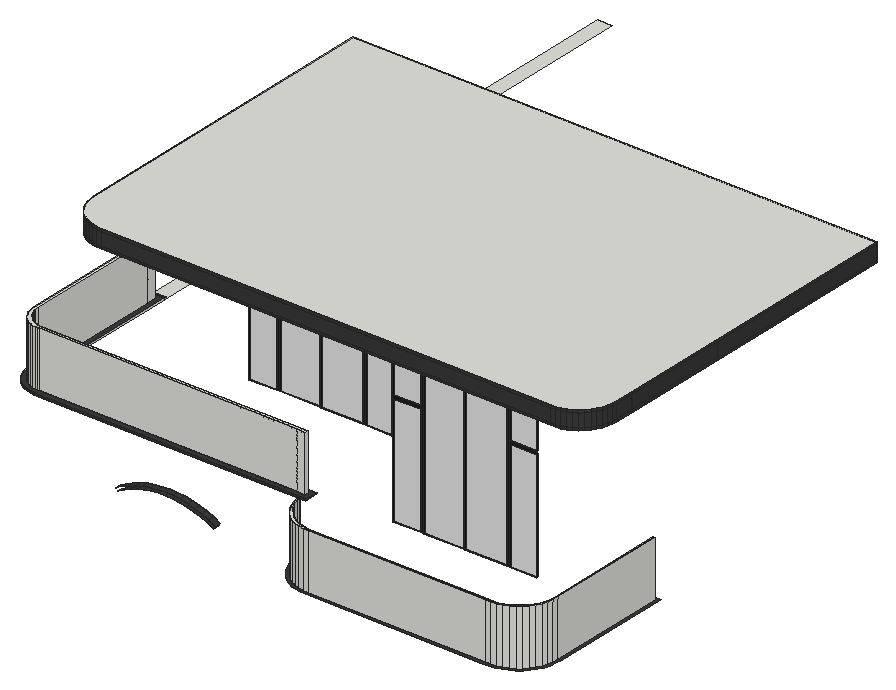
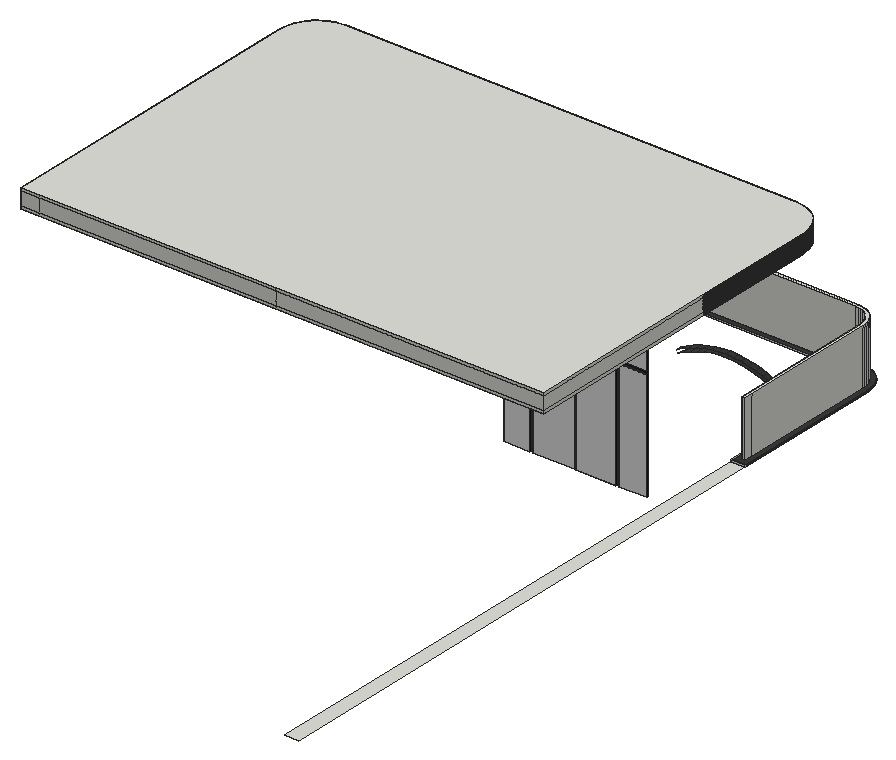
# SketchUp Ruby script. Lengths in inches.
U = 1.inch
M = Sketchup.active_model
def pt(a) = Geom::Point3d.new(a.map { |v| v * U })
def face(e, loops, mat)
  f = e.add_face(loops[0].map { |a| pt(a) })
  loops[1..].each { |l| e.add_face(l.map { |a| pt(a) }).erase! }
  f.material = f.back_material = mat if mat
  f
end
# faces: each face lists its corners as indices into pts; further lists are holes
def faces(e, pts, list, mat = nil) = list.each { |f| face(e, (f[0].is_a?(Array) ? f : [f]).map { |l| l.map { |i| pts[i] } }, mat) }
# xy, xz, yz: faces in a plane at the given z, y or x. An outline is a flat list of corners, or four numbers for a rectangle; further outlines are holes
def ring(l) = l.size == 4 ? [[l[0], l[1]], [l[2], l[1]], [l[2], l[3]], [l[0], l[3]]] : l.each_slice(2).to_a
def flat(e, list, mat, &to3) = list.each { |f| face(e, (f[0].is_a?(Array) ? f : [f]).map { |l| ring(l).map { |u, v| to3.(u, v) } }, mat) }
def xy(e, z, list, mat = nil) = flat(e, list, mat) { |x, y| [x, y, z] }
def xz(e, y, list, mat = nil) = flat(e, list, mat) { |x, z| [x, y, z] }
def yz(e, x, list, mat = nil) = flat(e, list, mat) { |y, z| [x, y, z] }
def lines(e, pts, list) = list.each { |a, b| e.add_line(pt(pts[a]), pt(pts[b])) }
# prism: a flat outline (further loops are holes) pulled along v
def prism(e, loops, v, mat = nil)
  f = face(e, loops, mat); d = Geom::Vector3d.new(v.map { |x| x * U })
  f.pushpull(f.normal.samedirection?(d) ? d.length : -d.length)
end
def box(e, o, s, mat = nil) = prism(e, [[o, [o[0] + s[0], o[1], o[2]], [o[0] + s[0], o[1] + s[1], o[2]], [o[0], o[1] + s[1], o[2]]]], [0, 0, s[2]], mat)
def at(x, y, z, deg = 0) = Geom::Transformation.translation(pt([x, y, z])) * Geom::Transformation.rotation(ORIGIN, Z_AXIS, deg.degrees)
def axes(o, x, y, z) = Geom::Transformation.new([*x, 0, *y, 0, *z, 0, *pt(o).to_a, 1])
def part(name) = M.definitions.add(name)
# library, detail: a bought-in or finely detailed component or shape, given as its bounding box
def library(name, o, s) = part(name).tap { |d| box(d.entities, o, s) }
def detail(e, o, s) = box(e.add_group.entities, o, s)
def put(e, d, t, mat = nil) = e.add_instance(d, t).tap { |i| i.material = mat if mat }
def group(e, t, mat = nil) = e.add_group.tap { |g| g.transformation = t; g.material = mat if mat }.entities
root = M.entities
M.materials.add("[Color M07]").color = [58, 58, 58]
M.materials.add("[Color M08]").color = [30, 30, 30]
M.materials.add("[Mirror 02]").color = [229, 229, 229]
xy(root,265.57,[[216.74,2.48,213.39,2.7,210.15,3.35,207.02,4.41,204.06,5.87,201.31,7.71,198.82,9.89,196.65,12.37,194.81,15.12,193.35,18.08,192.29,21.21,191.64,24.45,191.57,25.58,192.97,25.58,193.03,24.64,193.64,21.57,194.64,18.62,196.02,15.82,197.76,13.22,199.8125,10.875,202.16,8.82,204.76,7.08,207.56,5.7,210.51,4.7,213.57,4.09,216.79,3.88,331.6,3.88,335.01,3.93,338.19,4.4,341.28,5.31,344.22,6.62,346.96,8.3125,349.44,10.36,351.62,12.73,353.46,15.37,354.93,18.23,356,21.26,356.64,24.41,356.87,27.73,356.87,106.25,358.27,106.25,358.27,27.68,358.03,24.23,357.34,20.89,356.21,17.68,354.66,14.64,352.71,11.85,350.4,9.35,347.77,7.18,344.875,5.38,341.77,3.99,338.5,3.04,335.125,2.53,331.61,2.48],[189.6875,27.75,195,27.75,194.98,28.1]])
xy(root,265.57,[[[216.67,0.3125,331.63,0.3125,335.3,0.36,338.96,0.91,342.52,1.95,345.9,3.46,349.04,5.41,351.89,7.77,354.4,10.49,356.52,13.52,358.21,16.82,359.44,20.31,360.1875,23.93,360.4375,27.61,360.4375,108.42,354.7,108.42,354.7,27.8,354.49,24.71,353.9,21.85,352.93,19.09,351.59,16.49,349.92,14.09,347.94,11.94,345.6875,10.08,343.2,8.54,340.53,7.35,337.73,6.53,334.84,6.09,331.59,6.05,216.86,6.05,213.86,6.25,211.07,6.8,208.39,7.71,205.84,8.97,203.48,10.54,201.35,12.41,199.48,14.55,197.91,16.91,196.65,19.45,195.74,22.14,195.1875,24.92,195,27.75,189.6875,27.75,189.25,27.72,189.48,24.17,190.18,20.65,191.34,17.25,192.93,14.03,194.92,11.05,197.29,8.35,199.98,5.98,202.97,3.99,206.1875,2.4,209.59,1.25,213.11,0.55],[216.74,2.48,213.39,2.7,210.15,3.35,207.02,4.41,204.06,5.87,201.31,7.71,198.82,9.89,196.65,12.37,194.81,15.12,193.35,18.08,192.29,21.21,191.64,24.45,191.57,25.58,192.97,25.58,193.03,24.64,193.64,21.57,194.64,18.62,196.02,15.82,197.76,13.22,199.8125,10.875,202.16,8.82,204.76,7.08,207.56,5.7,210.51,4.7,213.57,4.09,216.79,3.88,331.6,3.88,335.01,3.93,338.19,4.4,341.28,5.31,344.22,6.62,346.96,8.3125,349.44,10.36,351.62,12.73,353.46,15.37,354.93,18.23,356,21.26,356.64,24.41,356.87,27.73,356.87,106.25,358.27,106.25,358.27,27.68,358.03,24.23,357.34,20.89,356.21,17.68,354.66,14.64,352.71,11.85,350.4,9.35,347.77,7.18,344.875,5.38,341.77,3.99,338.5,3.04,335.125,2.53,331.61,2.48]]],"[Color M07]")
xy(root,266.52,[[205.38,85.4375,223.05,86.25],[225.05,85.4375,250.97,86.25],[251.97,85.4375,278.89,86.25],[280.89,85.4375,298.16,86.25],[56.75,154.4375,74.42,155.25],
  [76.42,154.4375,102.34,155.25],[103.34,154.4375,130.27,155.25],[132.27,154.4375,149.53,155.25]],"[Color M08]")
xy(root,300,[[0,145.57,9,146.28],[0,146.28,9,507.75]])
xy(root,301.0625,[[18.77,31.13,16.92,31.25,14.92,31.65,12.99,32.3,11.16,33.21,9.47,34.34,7.93,35.68,6.59,37.22,5.46,38.91,4.55,40.74,3.9,42.67,3.5,44.67,3.38,46.52,3.38,142.2,5.62,142.2,5.62,46.89,5.75,44.97,6.09,43.26,6.65,41.61,7.42,40.05,8.39,38.6,9.54,37.29,10.85,36.14,12.3,35.17,13.86,34.4,15.51,33.84,17.22,33.5,19.14,33.37,191.62,33.37,191.62,31.13],[0,145.57,9,146.28]])
xy(root,301.0625,[[[18.66,27.75,195,27.75,195,36.75,19.25,36.75,17.66,36.85,16.39,37.11,15.15,37.53,13.99,38.1,12.91,38.82,11.93,39.68,11.07,40.66,10.35,41.74,9.78,42.9,9.36,44.14,9.1,45.41,9,47,9,145.57,0,145.57,0,46.41,0.14,44.23,0.63,41.8,1.43,39.45,2.52,37.22,3.9,35.16,5.54,33.29,7.41,31.65,9.47,30.27,11.7,29.18,14.05,28.38,16.48,27.89],[18.77,31.13,16.92,31.25,14.92,31.65,12.99,32.3,11.16,33.21,9.47,34.34,7.93,35.68,6.59,37.22,5.46,38.91,4.55,40.74,3.9,42.67,3.5,44.67,3.38,46.52,3.38,142.2,5.62,142.2,5.62,46.89,5.75,44.97,6.09,43.26,6.65,41.61,7.42,40.05,8.39,38.6,9.54,37.29,10.85,36.14,12.3,35.17,13.86,34.4,15.51,33.84,17.22,33.5,19.14,33.37,191.62,33.37,191.62,31.13]]],"[Color M07]")
xy(root,301.57,[[216.74,2.48,331.61,2.48,335.125,2.53,338.5,3.04,341.77,3.99,344.875,5.38,347.77,7.18,350.4,9.35,352.71,11.85,354.66,14.64,356.21,17.68,357.34,20.89,358.03,24.23,358.27,27.68,358.27,106.25,356.87,106.25,356.87,27.73,356.64,24.41,356,21.26,354.93,18.23,353.46,15.37,351.62,12.73,349.44,10.36,346.96,8.3125,344.22,6.62,341.28,5.31,338.19,4.4,335.01,3.93,331.6,3.88,216.79,3.88,213.57,4.09,210.51,4.7,207.56,5.7,204.76,7.08,202.16,8.82,199.8125,10.875,197.76,13.22,196.02,15.82,194.64,18.62,193.64,21.57,193.03,24.64,192.97,25.58,191.57,25.58,191.64,24.45,192.29,21.21,193.35,18.08,194.81,15.12,196.65,12.37,198.82,9.89,201.31,7.71,204.06,5.87,207.02,4.41,210.15,3.35,213.39,2.7]])
xy(root,337.0625,[[18.77,31.13,191.62,31.13,191.62,33.37,19.14,33.37,17.22,33.5,15.51,33.84,13.86,34.4,12.3,35.17,10.85,36.14,9.54,37.29,8.39,38.6,7.42,40.05,6.65,41.61,6.09,43.26,5.75,44.97,5.62,46.89,5.62,142.2,3.38,142.2,3.38,46.52,3.5,44.67,3.9,42.67,4.55,40.74,5.46,38.91,6.59,37.22,7.93,35.68,9.47,34.34,11.16,33.21,12.99,32.3,14.92,31.65,16.92,31.25]])
xy(root,337.86,[[205.38,85.4375,223.05,86.25],[280.89,85.4375,298.16,86.25],[56.75,154.4375,74.42,155.25],[132.27,154.4375,149.53,155.25]],"[Color M08]")
xy(root,339.86,[[205.38,85.4375,223.05,86.25],[280.89,85.4375,298.16,86.25],[56.75,154.4375,74.42,155.25],[132.27,154.4375,149.53,155.25]],"[Color M08]")
xy(root,363.92,[[205.38,85.4375,223.05,86.25],[225.05,85.4375,250.97,86.25],[251.97,85.4375,278.89,86.25],[280.89,85.4375,298.16,86.25],[56.75,154.4375,74.42,155.25],
  [76.42,154.4375,102.34,155.25],[103.34,154.4375,130.27,155.25],[132.27,154.4375,149.53,155.25]],"[Color M08]")
xy(root,366.4375,[[202.87,87.8125,300.68,94.4375],[54.24,156.8125,152.05,163.4375]])
xy(root,366.4375,[[202.87,85.4375,300.68,87.8125],[54.24,154.4375,152.05,156.8125]],"[Color M08]")
xy(root,384,[[45,49.4375,41.87,49.64,38.79,50.26,35.82,51.26,33,52.65,30.39,54.4,28.03,56.47,25.96,58.83,24.22,61.4375,22.83,64.25,21.82,67.23,21.21,70.3,21,73.4375,21,154.4375,35.42,154.4375,35.42,73.4375,35.5,72.1875,35.75,70.96,36.15,69.77,36.7,68.65,37.4,67.61,38.23,66.66,39.17,65.84,40.21,65.14,41.33,64.59,42.52,64.18,43.75,63.94,45,63.86,336,63.86,337.25,63.94,338.48,64.18,339.67,64.59,340.79,65.14,341.83,65.84,342.77,66.66,343.6,67.61,344.3,68.65,344.85,69.77,345.25,70.96,345.5,72.1875,345.58,73.4375,345.58,98.26,346.25,99.62,347.22,102.47,347.8,105.42,348,108.42,348,154.4375,360,154.4375,360,73.4375,359.79,70.3,359.18,67.23,358.17,64.25,356.78,61.4375,355.04,58.83,352.97,56.47,350.61,54.4,348,52.65,345.18,51.26,342.21,50.26,339.13,49.64,336,49.4375],[45,69.08,44.43,69.12,43.875,69.23,43.33,69.41,42.82,69.67,42.35,69.98,41.92,70.36,41.55,70.79,41.23,71.26,40.98,71.77,40.79,72.3125,40.68,72.87,40.65,73.4375,40.65,154.4375,185.6875,154.4375,185.6875,85.4375,325.02,85.4375,328.02,85.63,330.97,86.22,333.82,87.1875,336.51,88.52,339,90.18,339.01,90.1875,340.35,91.36,340.35,73.4375,340.32,72.87,340.21,72.3125,340.02,71.77,339.77,71.26,339.45,70.79,339.08,70.36,338.65,69.98,338.18,69.67,337.67,69.41,337.125,69.23,336.57,69.12,336,69.08],[185.6875,85.4375,194.6875,94.4375],[194.6875,85.4375,325.02,85.4375,328.02,85.63,330.97,86.22,333.82,87.1875,336.51,88.52,339,90.18,339,108.42,338.88,106.59,338.52,104.8,337.9375,103.07,337.13,101.43,336.11,99.91,334.91,98.53,333.53,97.33,332.01,96.31,330.37,95.5,328.64,94.91,326.85,94.56,325.02,94.4375,194.6875,94.4375],[339,90.18,339.01,90.1875,340.35,91.36,341.27,92.17,343.25,94.43,344.92,96.93,345.58,98.26,346.25,99.62,347.22,102.47,347.8,105.42,348,108.42,348,154.4375,339,154.4375],
  [185.6875,94.4375,194.6875,154.4375],[194.6875,94.4375,194.6875,214.4375,339,214.4375,339,108.42,338.88,106.59,338.52,104.8,337.9375,103.07,337.13,101.43,336.11,99.91,334.91,98.53,333.53,97.33,332.01,96.31,330.37,95.5,328.64,94.91,326.85,94.56,325.02,94.4375],[21,154.4375,21,283.4375,185.6875,283.4375,185.6875,274.4375,30,274.4375,30,163.4375,185.6875,163.4375,185.6875,154.4375],[185.6875,154.4375,194.6875,223.4375],[339,154.4375,348,214.4375],
  [348,154.4375,360,214.4375],[30,163.4375,185.6875,274.4375],[194.6875,214.4375,348,223.4375],[348,214.4375,360,223.4375],[185.6875,223.4375,194.6875,283.4375],
  [194.6875,223.4375,348,283.4375],[348,223.4375,360,283.4375]])
xy(root,385.5,[[45,49.4375,41.87,49.64,38.79,50.26,35.82,51.26,33,52.65,30.39,54.4,28.03,56.47,25.96,58.83,24.22,61.4375,22.83,64.25,21.82,67.23,21.21,70.3,21,73.4375,21,283.4375,360,283.4375,360,73.4375,359.79,70.3,359.18,67.23,358.17,64.25,356.78,61.4375,355.04,58.83,352.97,56.47,350.61,54.4,348,52.65,345.18,51.26,342.21,50.26,339.13,49.64,336,49.4375]])
xy(root,386.9375,[[45,63.86,43.75,63.94,42.52,64.18,41.33,64.59,40.21,65.14,39.17,65.84,38.23,66.66,37.4,67.61,36.7,68.65,36.15,69.77,35.75,70.96,35.5,72.1875,35.42,73.4375,35.42,154.4375,40.65,154.4375,40.65,73.4375,40.68,72.87,40.79,72.3125,40.98,71.77,41.23,71.26,41.55,70.79,41.92,70.36,42.35,69.98,42.82,69.67,43.33,69.41,43.875,69.23,44.43,69.12,45,69.08,336,69.08,336.57,69.12,337.125,69.23,337.67,69.41,338.18,69.67,338.65,69.98,339.08,70.36,339.45,70.79,339.77,71.26,340.02,71.77,340.21,72.3125,340.32,72.87,340.35,73.4375,340.35,91.36,341.27,92.17,343.25,94.43,344.92,96.93,345.58,98.26,345.58,73.4375,345.5,72.1875,345.25,70.96,344.85,69.77,344.3,68.65,343.6,67.61,342.77,66.66,341.83,65.84,340.79,65.14,339.67,64.59,338.48,64.18,337.25,63.94,336,63.86]])
xy(root,394.3125,[[45,49.4375,41.87,49.64,38.79,50.26,35.82,51.26,33,52.65,30.39,54.4,28.03,56.47,25.96,58.83,24.22,61.4375,22.83,64.25,21.82,67.23,21.21,70.3,21,73.4375,21,283.4375,360,283.4375,360,73.4375,359.79,70.3,359.18,67.23,358.17,64.25,356.78,61.4375,355.04,58.83,352.97,56.47,350.61,54.4,348,52.65,345.18,51.26,342.21,50.26,339.13,49.64,336,49.4375]])
xy(root,396,[[45,49.4375,336,49.4375,339.13,49.64,342.21,50.26,345.18,51.26,348,52.65,350.61,54.4,352.97,56.47,355.04,58.83,356.78,61.4375,358.17,64.25,359.18,67.23,359.79,70.3,360,73.4375,360,283.4375,21,283.4375,21,73.4375,21.21,70.3,21.82,67.23,22.83,64.25,24.22,61.4375,25.96,58.83,28.03,56.47,30.39,54.4,33,52.65,35.82,51.26,38.79,50.26,41.87,49.64]])
xz(root,2.48,[[216.74,265.57,331.61,301.57]])
xz(root,3.88,[[216.79,265.57,331.6,301.57]])
xz(root,25.58,[[191.57,265.57,192.97,301.57]])
xz(root,27.75,[[18.66,300,195,301.0625]],"[Color M07]")
xz(root,31.13,[[18.77,301.0625,18.96,337.0625],[18.96,301.0625,186,337.0625],[186,301.0625,191.62,337.0625]])
xz(root,33.37,[[19.14,301.0625,186,337.0625],[186,301.0625,191.62,337.0625]])
xz(root,36.75,[[18.96,300,195,301.0625]])
xz(root,49.4375,[[45,384,336,385.5],[45,385.5,336,394.3125],[45,394.3125,336,396]],"[Color M07]")
xz(root,63.86,[[45,384,336,386.9375]])
xz(root,69.08,[[45,384,336,386.9375]])
xz(root,85.4375,[[223.05,266.52,225.05,363.92],[250.97,266.52,251.97,363.92],[278.89,266.52,280.89,363.92],[205.38,337.86,223.05,339.86],[280.89,337.86,298.16,339.86]],"[Color M08]")
xz(root,86.25,[[205.38,266.52,223.05,337.86],[225.05,266.52,250.97,363.92],[251.97,266.52,278.89,363.92],[280.89,266.52,298.16,337.86],[205.38,339.86,223.05,363.92],
  [280.89,339.86,298.16,363.92]],"[Mirror 02]")
xz(root,106.25,[[356.87,265.57,358.27,301.57]])
xz(root,142.2,[[3.38,301.0625,5.62,337.0625]])
xz(root,145.57,[[0,300,9,301.0625]])
xz(root,146.28,[[0,300,9,301.0625]])
xz(root,154.4375,[[35.42,384,40.65,386.9375]])
xz(root,154.4375,[[74.42,266.52,76.42,363.92],[102.34,266.52,103.34,363.92],[130.27,266.52,132.27,363.92],[56.75,337.86,74.42,339.86],[132.27,337.86,149.53,339.86]],"[Color M08]")
xz(root,155.25,[[56.75,266.52,74.42,337.86],[76.42,266.52,102.34,363.92],[103.34,266.52,130.27,363.92],[132.27,266.52,149.53,337.86],[56.75,339.86,74.42,363.92],
  [132.27,339.86,149.53,363.92]],"[Mirror 02]")
xz(root,283.4375,[[21,384,194.6875,385.5],[194.6875,384,348,385.5],[348,384,360,385.5],[21,385.5,194.6875,394.3125],[194.6875,385.5,348,394.3125],
  [348,385.5,360,394.3125],[21,394.3125,194.6875,396],[194.6875,394.3125,348,396],[348,394.3125,360,396]])
yz(root,0,[[145.57,300,146.28,301.0625]])
yz(root,0,[[46.41,300,145.57,301.0625]],"[Color M07]")
yz(root,3.38,[[46.52,301.0625,46.71,337.0625],[46.71,301.0625,136.57,337.0625],[136.57,301.0625,142.2,337.0625]])
yz(root,5.62,[[46.89,301.0625,136.57,337.0625],[136.57,301.0625,142.2,337.0625]])
yz(root,9,[[46.71,300,145.57,301.0625],[145.57,300,146.28,301.0625]])
yz(root,21,[[154.4375,384,283.4375,385.5],[154.4375,385.5,283.4375,394.3125],[154.4375,394.3125,283.4375,396]])
yz(root,21,[[73.4375,384,154.4375,385.5],[73.4375,385.5,154.4375,394.3125],[73.4375,394.3125,154.4375,396]],"[Color M07]")
yz(root,35.42,[[73.4375,384,140.02,386.9375],[140.02,384,154.4375,386.9375]])
yz(root,40.65,[[73.4375,384,140.02,386.9375],[140.02,384,154.4375,386.9375]])
yz(root,56.75,[[154.4375,266.52,155.25,337.86],[154.4375,339.86,155.25,363.92]],"[Color M08]")
yz(root,74.42,[[154.4375,266.52,155.25,337.86],[154.4375,339.86,155.25,363.92]],"[Color M08]")
yz(root,76.42,[[154.4375,266.52,155.25,363.92]],"[Color M08]")
yz(root,102.34,[[154.4375,266.52,155.25,363.92]],"[Color M08]")
yz(root,103.34,[[154.4375,266.52,155.25,363.92]],"[Color M08]")
yz(root,130.27,[[154.4375,266.52,155.25,363.92]],"[Color M08]")
yz(root,132.27,[[154.4375,266.52,155.25,337.86],[154.4375,339.86,155.25,363.92]],"[Color M08]")
yz(root,149.53,[[154.4375,266.52,155.25,337.86],[154.4375,339.86,155.25,363.92]],"[Color M08]")
yz(root,191.62,[[31.13,301.0625,33.37,337.0625]])
yz(root,195,[[27.75,300,36.75,301.0625]],"[Color M07]")
yz(root,205.38,[[85.4375,266.52,86.25,337.86],[85.4375,339.86,86.25,363.92]],"[Color M08]")
yz(root,223.05,[[85.4375,266.52,86.25,337.86],[85.4375,339.86,86.25,363.92]],"[Color M08]")
yz(root,225.05,[[85.4375,266.52,86.25,363.92]],"[Color M08]")
yz(root,250.97,[[85.4375,266.52,86.25,363.92]],"[Color M08]")
yz(root,251.97,[[85.4375,266.52,86.25,363.92]],"[Color M08]")
yz(root,278.89,[[85.4375,266.52,86.25,363.92]],"[Color M08]")
yz(root,280.89,[[85.4375,266.52,86.25,337.86],[85.4375,339.86,86.25,363.92]],"[Color M08]")
yz(root,298.16,[[85.4375,266.52,86.25,337.86],[85.4375,339.86,86.25,363.92]],"[Color M08]")
yz(root,340.35,[[73.4375,384,91.36,386.9375]])
yz(root,345.58,[[73.4375,384,98.26,386.9375]])
yz(root,356.87,[[27.73,265.57,106.25,301.57]])
yz(root,358.27,[[27.68,265.57,106.25,301.57]])
yz(root,360,[[73.4375,384,85.4375,385.5],[85.4375,384,154.4375,385.5],[154.4375,384,283.4375,385.5],[73.4375,385.5,85.4375,394.3125],[85.4375,385.5,154.4375,394.3125],
  [154.4375,385.5,283.4375,394.3125],[73.4375,394.3125,85.4375,396],[85.4375,394.3125,154.4375,396],[154.4375,394.3125,283.4375,396]],"[Color M07]")
p = [[75.74,27.75,265.51],[79.87,27.75,267.71],[79.87,24.0625,267.71],[75.74,24.0625,265.51],[134.09,27.75,267.71],[138.21,27.75,265.51],
  [138.21,24.0625,265.51],[134.09,24.0625,267.71],[213.39,2.7,265.57],[216.74,2.48,265.57],[216.74,2.48,301.57],[213.39,2.7,301.57],
  [331.61,2.48,265.57],[335.125,2.53,265.57],[335.125,2.53,301.57],[331.61,2.48,301.57],[338.5,3.04,265.57],[338.5,3.04,301.57],
  [210.15,3.35,265.57],[210.15,3.35,301.57],[341.77,3.99,265.57],[341.77,3.99,301.57],[207.02,4.41,265.57],[207.02,4.41,301.57],
  [216.79,3.88,265.57],[213.57,4.09,265.57],[213.57,4.09,301.57],[216.79,3.88,301.57],[335.01,3.93,265.57],[331.6,3.88,265.57],
  [331.6,3.88,301.57],[335.01,3.93,301.57],[338.19,4.4,265.57],[338.19,4.4,301.57],[344.875,5.38,265.57],[344.875,5.38,301.57],
  [210.51,4.7,265.57],[210.51,4.7,301.57],[204.06,5.87,265.57],[204.06,5.87,301.57],[341.28,5.31,265.57],[341.28,5.31,301.57],
  [207.56,5.7,265.57],[207.56,5.7,301.57],[344.22,6.62,265.57],[344.22,6.62,301.57],[347.77,7.18,265.57],[347.77,7.18,301.57],
  [204.76,7.08,265.57],[204.76,7.08,301.57],[201.31,7.71,265.57],[201.31,7.71,301.57],[346.96,8.3125,265.57],[346.96,8.3125,301.57],
  [202.16,8.82,265.57],[202.16,8.82,301.57],[350.4,9.35,265.57],[350.4,9.35,301.57],[198.82,9.89,265.57],[198.82,9.89,301.57],
  [349.44,10.36,265.57],[349.44,10.36,301.57],[199.8125,10.875,265.57],[199.8125,10.875,301.57],[352.71,11.85,265.57],[352.71,11.85,301.57],
  [196.65,12.37,265.57],[196.65,12.37,301.57],[351.62,12.73,265.57],[351.62,12.73,301.57],[197.76,13.22,265.57],[197.76,13.22,301.57],
  [354.66,14.64,265.57],[354.66,14.64,301.57],[194.81,15.12,265.57],[194.81,15.12,301.57],[353.46,15.37,265.57],[353.46,15.37,301.57],
  [196.02,15.82,265.57],[196.02,15.82,301.57],[356.21,17.68,265.57],[356.21,17.68,301.57],[193.35,18.08,265.57],[193.35,18.08,301.57],
  [354.93,18.23,265.57],[354.93,18.23,301.57],[194.64,18.62,265.57],[194.64,18.62,301.57],[357.34,20.89,265.57],[357.34,20.89,301.57],
  [192.29,21.21,265.57],[192.29,21.21,301.57],[356,21.26,265.57],[356,21.26,301.57],[193.64,21.57,265.57],[193.64,21.57,301.57],
  [358.03,24.23,265.57],[358.03,24.23,301.57],[191.64,24.45,265.57],[191.64,24.45,301.57],[356.64,24.41,265.57],[356.64,24.41,301.57],
  [193.03,24.64,265.57],[193.03,24.64,301.57],[358.27,27.68,265.57],[358.27,27.68,301.57],[356.87,27.73,265.57],[356.87,27.73,301.57],
  [191.57,25.58,265.57],[191.57,25.58,301.57],[192.97,25.58,265.57],[192.97,25.58,301.57],[78.97,27.75,269.5625],[74.71,27.75,267.29],
  [74.71,24.0625,267.29],[78.97,24.0625,269.5625],[139.25,27.75,267.29],[134.99,27.75,269.5625],[134.99,24.0625,269.5625],[139.25,24.0625,267.29],
  [84.15,27.75,269.59],[84.15,24.0625,269.59],[129.81,27.75,269.59],[129.81,24.0625,269.59],[83.39,27.75,271.51],[83.39,24.0625,271.51],
  [88.56,27.75,271.14],[88.56,24.0625,271.14],[125.4,27.75,271.14],[125.4,24.0625,271.14],[130.57,27.75,271.51],[130.57,24.0625,271.51],
  [93.07,27.75,272.36],[93.07,24.0625,272.36],[120.89,27.75,272.36],[120.89,24.0625,272.36],[87.95,27.75,273.11],[87.95,24.0625,273.11],
  [126.01,27.75,273.11],[126.01,24.0625,273.11],[97.66,27.75,273.24],[97.66,24.0625,273.24],[116.3,27.75,273.24],[116.3,24.0625,273.24],
  [92.61,27.75,274.37],[92.61,24.0625,274.37],[121.35,27.75,274.37],[121.35,24.0625,274.37],[102.31,27.75,273.76],[102.31,24.0625,273.76],
  [111.65,27.75,273.76],[111.65,24.0625,273.76],[106.98,27.75,273.9375],[106.98,24.0625,273.9375],[97.35,27.75,275.27],[97.35,24.0625,275.27],
  [116.6,27.75,275.27],[116.6,24.0625,275.27],[102.15,27.75,275.82],[102.15,24.0625,275.82],[111.81,27.75,275.82],[111.81,24.0625,275.82],
  [106.98,27.75,276],[106.98,24.0625,276],[16.48,27.91,301.0625],[16.48,27.91,300],[18.96,27.75,300],[18.96,27.75,301.0625],
  [18.66,27.75,300],[18.66,27.75,301.0625],[16.48,27.89,301.0625],[16.48,27.89,300],[14.05,28.38,301.0625],[14.05,28.38,300],
  [14.05,28.4,301.0625],[14.05,28.4,300],[11.7,29.19,301.0625],[11.7,29.19,300],[11.7,29.18,301.0625],[11.7,29.18,300],
  [9.48,30.29,301.0625],[9.48,30.29,300],[9.47,30.27,301.0625],[9.47,30.27,300],[7.41,31.65,301.0625],[7.41,31.65,300],
  [7.42,31.67,301.0625],[7.42,31.67,300],[9,30.61,300],[9,30.61,301.0625],[5.54,33.29,301.0625],[5.54,33.29,300],
  [5.55,33.3,301.0625],[5.55,33.3,300],[3.92,35.17,301.0625],[3.92,35.17,300],[3.9,35.16,301.0625],[3.9,35.16,300],
  [2.54,37.23,301.0625],[2.54,37.23,300],[2.52,37.22,301.0625],[2.52,37.22,300],[17.66,36.85,300],[17.66,36.85,301.0625],
  [19.25,36.75,301.0625],[19.25,36.75,300],[18.96,36.75,301.0625],[18.96,36.75,300],[17.66,36.84,300],[17.66,36.84,301.0625],
  [16.38,37.09,300],[16.38,37.09,301.0625],[16.39,37.11,300],[16.39,37.11,301.0625],[15.15,37.51,300],[15.15,37.51,301.0625],
  [15.15,37.53,300],[15.15,37.53,301.0625],[1.44,39.45,301.0625],[1.44,39.45,300],[1.43,39.45,301.0625],[1.43,39.45,300],
  [13.99,38.1,300],[13.99,38.1,301.0625],[13.98,38.08,300],[13.98,38.08,301.0625],[12.91,38.82,300],[12.91,38.82,301.0625],
  [14,38.09,301.0625],[14,38.09,300],[12.9,38.81,300],[12.9,38.81,301.0625],[11.93,39.68,300],[11.93,39.68,301.0625],
  [11.92,39.67,300],[11.92,39.67,301.0625],[0.63,41.8,301.0625],[0.63,41.8,300],[0.65,41.8,301.0625],[0.65,41.8,300],
  [11.07,40.66,300],[11.07,40.66,301.0625],[11.06,40.65,300],[11.06,40.65,301.0625],[10.33,41.73,300],[10.33,41.73,301.0625],
  [10.35,41.74,300],[10.35,41.74,301.0625],[9.78,42.9,300],[9.78,42.9,301.0625],[9.76,42.9,300],[9.76,42.9,301.0625],
  [0.14,44.23,301.0625],[0.14,44.23,300],[0.16,44.23,301.0625],[0.16,44.23,300],[9.34,44.13,300],[9.34,44.13,301.0625],
  [9.36,44.14,300],[9.36,44.14,301.0625],[9.1,45.41,300],[9.1,45.41,301.0625],[9.09,45.41,300],[9.09,45.41,301.0625],
  [0,46.71,301.0625],[0,46.71,300],[0.02,46.41,300],[0.02,46.41,301.0625],[0,46.41,301.0625],[0,46.41,300],
  [9,47,300],[9,47,301.0625],[9,46.71,300],[9,46.71,301.0625],[16.92,31.25,301.0625],[18.77,31.13,301.0625],
  [18.77,31.13,337.0625],[16.92,31.25,337.0625],[14.92,31.65,301.0625],[14.92,31.65,337.0625],[12.99,32.3,301.0625],[12.99,32.3,337.0625],
  [11.16,33.21,301.0625],[11.16,33.21,337.0625],[9.47,34.34,301.0625],[9.47,34.34,337.0625],[19.14,33.37,301.0625],[17.22,33.5,301.0625],
  [17.22,33.5,337.0625],[19.14,33.37,337.0625],[15.51,33.84,301.0625],[15.51,33.84,337.0625],[13.86,34.4,301.0625],[13.86,34.4,337.0625],
  [7.93,35.68,301.0625],[7.93,35.68,337.0625],[12.3,35.17,301.0625],[12.3,35.17,337.0625],[10.85,36.14,301.0625],[10.85,36.14,337.0625],
  [6.59,37.22,301.0625],[6.59,37.22,337.0625],[9.54,37.29,301.0625],[9.54,37.29,337.0625],[5.46,38.91,301.0625],[5.46,38.91,337.0625],
  [8.39,38.6,301.0625],[8.39,38.6,337.0625],[7.42,40.05,301.0625],[7.42,40.05,337.0625],[4.55,40.74,301.0625],[4.55,40.74,337.0625],
  [6.65,41.61,301.0625],[6.65,41.61,337.0625],[3.9,42.67,301.0625],[3.9,42.67,337.0625],[6.09,43.26,301.0625],[6.09,43.26,337.0625],
  [3.5,44.67,301.0625],[3.5,44.67,337.0625],[5.75,44.97,301.0625],[5.75,44.97,337.0625],[3.38,46.52,301.0625],[3.38,46.52,337.0625],
  [5.62,46.89,301.0625],[5.62,46.89,337.0625],[45,49.4375,384],[45,49.4375,385.5],[41.87,49.64,385.5],[41.87,49.64,384],
  [339.13,49.64,384],[339.13,49.64,385.5],[336,49.4375,385.5],[336,49.4375,384],[38.79,50.26,385.5],[38.79,50.26,384],
  [342.21,50.26,384],[342.21,50.26,385.5],[35.82,51.26,385.5],[35.82,51.26,384],[345.18,51.26,384],[345.18,51.26,385.5],
  [33,52.65,385.5],[33,52.65,384],[348,52.65,384],[348,52.65,385.5],[30.39,54.4,385.5],[30.39,54.4,384],
  [350.61,54.4,384],[350.61,54.4,385.5],[28.03,56.47,385.5],[28.03,56.47,384],[352.97,56.47,384],[352.97,56.47,385.5],
  [25.96,58.83,385.5],[25.96,58.83,384],[355.04,58.83,384],[355.04,58.83,385.5],[24.22,61.4375,385.5],[24.22,61.4375,384],
  [356.78,61.4375,384],[356.78,61.4375,385.5],[22.83,64.25,385.5],[22.83,64.25,384],[358.17,64.25,384],[358.17,64.25,385.5],
  [43.75,63.94,384],[42.52,64.18,384],[42.52,64.18,386.9375],[43.75,63.94,386.9375],[45,63.86,384],[45,63.86,386.9375],
  [337.25,63.94,384],[336,63.86,384],[336,63.86,386.9375],[337.25,63.94,386.9375],[338.48,64.18,384],[338.48,64.18,386.9375],
  [41.33,64.59,384],[41.33,64.59,386.9375],[339.67,64.59,384],[339.67,64.59,386.9375],[21.82,67.23,385.5],[21.82,67.23,384],
  [359.18,67.23,384],[359.18,67.23,385.5],[40.21,65.14,384],[40.21,65.14,386.9375],[340.79,65.14,384],[340.79,65.14,386.9375],
  [39.17,65.84,384],[39.17,65.84,386.9375],[341.83,65.84,384],[341.83,65.84,386.9375],[38.23,66.66,384],[38.23,66.66,386.9375],
  [342.77,66.66,384],[342.77,66.66,386.9375],[37.4,67.61,384],[37.4,67.61,386.9375],[343.6,67.61,384],[343.6,67.61,386.9375],
  [21.21,70.3,385.5],[21.21,70.3,384],[359.79,70.3,384],[359.79,70.3,385.5],[36.7,68.65,384],[36.7,68.65,386.9375],
  [344.3,68.65,384],[344.3,68.65,386.9375],[36.15,69.77,384],[36.15,69.77,386.9375],[344.85,69.77,384],[344.85,69.77,386.9375],
  [43.875,69.23,384],[44.43,69.12,384],[44.43,69.12,386.9375],[43.875,69.23,386.9375],[45,69.08,384],[45,69.08,386.9375],
  [336,69.08,384],[336.57,69.12,384],[336.57,69.12,386.9375],[336,69.08,386.9375],[337.125,69.23,384],[337.125,69.23,386.9375],
  [43.33,69.41,384],[43.33,69.41,386.9375],[337.67,69.41,384],[337.67,69.41,386.9375],[42.82,69.67,384],[42.82,69.67,386.9375],
  [338.18,69.67,384],[338.18,69.67,386.9375],[42.35,69.98,384],[42.35,69.98,386.9375],[338.65,69.98,384],[338.65,69.98,386.9375],
  [35.75,70.96,384],[35.75,70.96,386.9375],[345.25,70.96,384],[345.25,70.96,386.9375],[41.92,70.36,384],[41.92,70.36,386.9375],
  [339.08,70.36,384],[339.08,70.36,386.9375],[21,73.4375,385.5],[21,73.4375,384],[360,73.4375,384],[360,73.4375,385.5],
  [41.55,70.79,384],[41.55,70.79,386.9375],[339.45,70.79,384],[339.45,70.79,386.9375],[41.23,71.26,384],[41.23,71.26,386.9375],
  [339.77,71.26,384],[339.77,71.26,386.9375],[35.5,72.1875,384],[35.5,72.1875,386.9375],[345.5,72.1875,384],[345.5,72.1875,386.9375],
  [40.98,71.77,384],[40.98,71.77,386.9375],[340.02,71.77,384],[340.02,71.77,386.9375],[40.79,72.3125,384],[40.79,72.3125,386.9375],
  [340.21,72.3125,384],[340.21,72.3125,386.9375],[35.42,73.4375,384],[35.42,73.4375,386.9375],[345.58,73.4375,384],[345.58,73.4375,386.9375],
  [40.68,72.87,384],[40.68,72.87,386.9375],[340.32,72.87,384],[340.32,72.87,386.9375],[40.65,73.4375,384],[40.65,73.4375,386.9375],
  [340.35,73.4375,384],[340.35,73.4375,386.9375],[340.35,91.36,384],[341.27,92.17,384],[341.27,92.17,386.9375],[340.35,91.36,386.9375],
  [343.25,94.43,384],[343.25,94.43,386.9375],[344.92,96.93,384],[344.92,96.93,386.9375],[345.58,98.26,384],[345.58,98.26,386.9375],
  [41.87,49.64,394.3125],[45,49.4375,394.3125],[336,49.4375,394.3125],[339.13,49.64,394.3125],[38.79,50.26,394.3125],[342.21,50.26,394.3125],
  [35.82,51.26,394.3125],[345.18,51.26,394.3125],[33,52.65,394.3125],[348,52.65,394.3125],[30.39,54.4,394.3125],[350.61,54.4,394.3125],
  [28.03,56.47,394.3125],[352.97,56.47,394.3125],[25.96,58.83,394.3125],[355.04,58.83,394.3125],[24.22,61.4375,394.3125],[356.78,61.4375,394.3125],
  [22.83,64.25,394.3125],[358.17,64.25,394.3125],[21.82,67.23,394.3125],[359.18,67.23,394.3125],[21.21,70.3,394.3125],[359.79,70.3,394.3125],
  [21,73.4375,394.3125],[360,73.4375,394.3125],[45,49.4375,396],[41.87,49.64,396],[339.13,49.64,396],[336,49.4375,396],
  [38.79,50.26,396],[342.21,50.26,396],[35.82,51.26,396],[345.18,51.26,396],[33,52.65,396],[348,52.65,396],
  [30.39,54.4,396],[350.61,54.4,396],[28.03,56.47,396],[352.97,56.47,396],[25.96,58.83,396],[355.04,58.83,396],
  [24.22,61.4375,396],[356.78,61.4375,396],[22.83,64.25,396],[358.17,64.25,396],[21.82,67.23,396],[359.18,67.23,396],
  [21.21,70.3,396],[359.79,70.3,396],[21,73.4375,396],[360,73.4375,396],[194.6875,154.4375,384],[194.6875,154.4375,396],
  [348,154.4375,384],[348,154.4375,396],[194.6875,85.4375,384],[194.6875,85.4375,396],[348,85.4375,384],[348,85.4375,396],
  [298.16,86.25,339.86],[298.23,86.25,339.86],[149.53,155.25,339.86],[149.6,155.25,339.86]]
faces(root,p,[[0,1,2,3],[4,5,6,7],[112,113,114,115],[116,117,118,119],[1,120,121,2],[122,4,7,123],[124,112,115,125],[120,126,127,121],
  [128,122,123,129],[117,130,131,118],[126,132,133,127],[134,128,129,135],[136,124,125,137],[130,138,139,131],[132,140,141,133],[142,134,135,143],
  [144,136,137,145],[138,146,147,139],[140,148,149,141],[150,142,143,151],[148,152,153,149],[152,150,151,153],[154,144,145,155],[146,156,157,147],
  [158,154,155,159],[156,160,161,157],[162,158,159,163],[160,162,163,161],[168,169,170,171],[171,170,172,173],[173,172,178,179],[179,178,182,183],
  [183,182,184,185],[185,184,190,191],[191,190,196,197],[197,196,200,201],[201,200,220,221],[221,220,236,237],[237,236,252,253],[253,252,268,269],
  [326,327,328,329],[330,331,332,333],[329,328,334,335],[336,337,331,330],[335,334,338,339],[340,341,337,336],[339,338,342,343],[344,345,341,340],
  [343,342,346,347],[348,349,345,344],[347,346,350,351],[352,353,349,348],[351,350,354,355],[356,357,353,352],[355,354,358,359],[360,361,357,356],
  [359,358,362,363],[364,365,361,360],[363,362,382,383],[384,385,365,364],[383,382,402,403],[404,405,385,384],[403,402,446,447],[448,449,405,404],
  [492,328,327,493],[494,332,331,495],[496,334,328,492],[495,331,337,497],[498,338,334,496],[497,337,341,499],[500,342,338,498],[499,341,345,501],
  [502,346,342,500],[501,345,349,503],[504,350,346,502],[503,349,353,505],[506,354,350,504],[505,353,357,507],[508,358,354,506],[507,357,361,509],
  [510,362,358,508],[509,361,365,511],[512,382,362,510],[511,365,385,513],[514,402,382,512],[513,385,405,515],[516,446,402,514],[515,405,449,517],
  [518,519,492,493],[520,521,494,495],[519,522,496,492],[523,520,495,497],[522,524,498,496],[525,523,497,499],[524,526,500,498],[527,525,499,501],
  [526,528,502,500],[529,527,501,503],[528,530,504,502],[531,529,503,505],[530,532,506,504],[533,531,505,507],[532,534,508,506],[535,533,507,509],
  [534,536,510,508],[537,535,509,511],[536,538,512,510],[539,537,511,513],[538,540,514,512],[541,539,513,515],[540,542,516,514],[543,541,515,517]],"[Color M07]")
faces(root,p,[[8,9,10,11],[12,13,14,15],[13,16,17,14],[18,8,11,19],[16,20,21,17],[22,18,19,23],[24,25,26,27],[28,29,30,31],
  [32,28,31,33],[20,34,35,21],[25,36,37,26],[38,22,23,39],[40,32,33,41],[36,42,43,37],[44,40,41,45],[34,46,47,35],
  [42,48,49,43],[50,38,39,51],[52,44,45,53],[48,54,55,49],[46,56,57,47],[58,50,51,59],[60,52,53,61],[54,62,63,55],
  [56,64,65,57],[66,58,59,67],[68,60,61,69],[62,70,71,63],[64,72,73,65],[74,66,67,75],[76,68,69,77],[70,78,79,71],
  [72,80,81,73],[82,74,75,83],[84,76,77,85],[78,86,87,79],[80,88,89,81],[90,82,83,91],[92,84,85,93],[86,94,95,87],
  [88,96,97,89],[98,90,91,99],[100,92,93,101],[94,102,103,95],[96,104,105,97],[106,100,101,107],[108,98,99,109],[102,110,111,103],
  [164,165,166,167],[174,175,165,164],[176,177,175,174],[180,181,177,176],[186,187,188,181,180,189],[192,193,187,186],[194,195,193,192],[198,199,195,194],
  [202,203,204,205],[206,207,208,209],[209,208,210,211],[212,213,203,202],[211,210,214,215],[216,217,213,212],[218,219,199,198],[222,223,217,216],
  [215,214,224,225],[226,227,223,228,229,222],[225,224,230,231],[232,233,227,226],[231,230,234,235],[238,239,219,218],[240,241,233,232],[235,234,242,243],
  [243,242,244,245],[246,247,241,240],[248,249,247,246],[245,244,250,251],[254,255,239,238],[251,250,256,257],[258,259,249,248],[260,261,259,258],
  [257,256,262,263],[264,265,266,255,254,267],[270,271,261,260],[263,262,272,273],[274,275,276,277],[278,274,277,279],[280,278,279,281],[282,280,281,283],
  [284,282,283,285],[286,287,288,289],[287,290,291,288],[290,292,293,291],[294,284,285,295],[292,296,297,293],[296,298,299,297],[300,294,295,301],
  [298,302,303,299],[304,300,301,305],[302,306,307,303],[306,308,309,307],[310,304,305,311],[308,312,313,309],[314,310,311,315],[312,316,317,313],
  [318,314,315,319],[316,320,321,317],[322,318,319,323],[320,324,325,321],[366,367,368,369],[370,366,369,371],[372,373,374,375],[376,372,375,377],
  [367,378,379,368],[380,376,377,381],[378,386,387,379],[388,380,381,389],[386,390,391,387],[392,388,389,393],[390,394,395,391],[396,392,393,397],
  [394,398,399,395],[400,396,397,401],[398,406,407,399],[408,400,401,409],[406,410,411,407],[412,408,409,413],[414,415,416,417],[415,418,419,416],
  [420,421,422,423],[421,424,425,422],[426,414,417,427],[424,428,429,425],[430,426,427,431],[428,432,433,429],[434,430,431,435],[432,436,437,433],
  [410,438,439,411],[440,412,413,441],[442,434,435,443],[436,444,445,437],[450,442,443,451],[444,452,453,445],[454,450,451,455],[452,456,457,453],
  [438,458,459,439],[460,440,441,461],[462,454,455,463],[456,464,465,457],[466,462,463,467],[464,468,469,465],[458,470,471,459],[472,460,461,473],
  [474,466,467,475],[468,476,477,469],[478,474,475,479],[476,480,481,477],[482,483,484,485],[483,486,487,484],[486,488,489,487],[488,490,491,489]])
lines(root,p,[[544,545],[546,547],[548,549],[550,551],[552,553],[554,555]])
